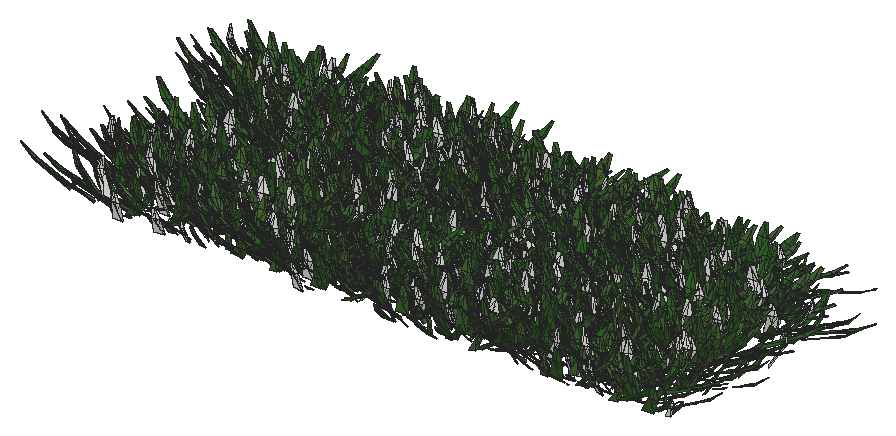
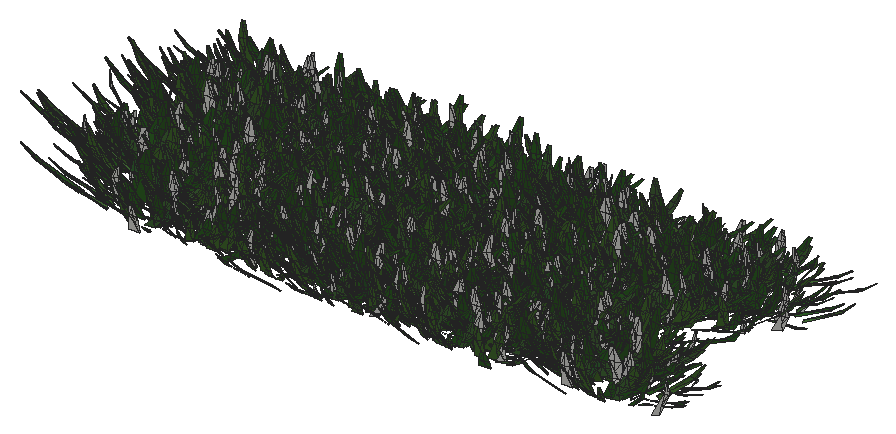
# SketchUp Ruby script. Lengths in inches.
U = 1.inch
M = Sketchup.active_model
def pt(a) = Geom::Point3d.new(a.map { |v| v * U })
def face(e, loops, mat)
  f = e.add_face(loops[0].map { |a| pt(a) })
  loops[1..].each { |l| e.add_face(l.map { |a| pt(a) }).erase! }
  f.material = f.back_material = mat if mat
  f
end
# faces: each face lists its corners as indices into pts; further lists are holes
def faces(e, pts, list, mat = nil) = list.each { |f| face(e, (f[0].is_a?(Array) ? f : [f]).map { |l| l.map { |i| pts[i] } }, mat) }
# xy, xz, yz: faces in a plane at the given z, y or x. An outline is a flat list of corners, or four numbers for a rectangle; further outlines are holes
def ring(l) = l.size == 4 ? [[l[0], l[1]], [l[2], l[1]], [l[2], l[3]], [l[0], l[3]]] : l.each_slice(2).to_a
def flat(e, list, mat, &to3) = list.each { |f| face(e, (f[0].is_a?(Array) ? f : [f]).map { |l| ring(l).map { |u, v| to3.(u, v) } }, mat) }
def xy(e, z, list, mat = nil) = flat(e, list, mat) { |x, y| [x, y, z] }
def xz(e, y, list, mat = nil) = flat(e, list, mat) { |x, z| [x, y, z] }
def yz(e, x, list, mat = nil) = flat(e, list, mat) { |y, z| [x, y, z] }
def lines(e, pts, list) = list.each { |a, b| e.add_line(pt(pts[a]), pt(pts[b])) }
# prism: a flat outline (further loops are holes) pulled along v
def prism(e, loops, v, mat = nil)
  f = face(e, loops, mat); d = Geom::Vector3d.new(v.map { |x| x * U })
  f.pushpull(f.normal.samedirection?(d) ? d.length : -d.length)
end
def box(e, o, s, mat = nil) = prism(e, [[o, [o[0] + s[0], o[1], o[2]], [o[0] + s[0], o[1] + s[1], o[2]], [o[0], o[1] + s[1], o[2]]]], [0, 0, s[2]], mat)
def at(x, y, z, deg = 0) = Geom::Transformation.translation(pt([x, y, z])) * Geom::Transformation.rotation(ORIGIN, Z_AXIS, deg.degrees)
def axes(o, x, y, z) = Geom::Transformation.new([*x, 0, *y, 0, *z, 0, *pt(o).to_a, 1])
def part(name) = M.definitions.add(name)
# library, detail: a bought-in or finely detailed component or shape, given as its bounding box
def library(name, o, s) = part(name).tap { |d| box(d.entities, o, s) }
def detail(e, o, s) = box(e.add_group.entities, o, s)
def put(e, d, t, mat = nil) = e.add_instance(d, t).tap { |i| i.material = mat if mat }
def group(e, t, mat = nil) = e.add_group.tap { |g| g.transformation = t; g.material = mat if mat }.entities
root = M.entities
M.materials.add("Material82").color = [68, 110, 58]
M.materials.add("Material83").color = [48, 90, 38]
M.materials.add("Material84").color = [68, 110, 48]
M.materials.add("Material85").color = [48, 90, 48]
M.materials.add("Material86").color = [58, 110, 58]
M.materials.add("Material87").color = [58, 90, 38]
M.materials.add("Material88").color = [68, 100, 58]
M.materials.add("Material89").color = [48, 100, 38]
c1 = part("grass00")
p = [[-0.6875,0.15,0],[-0.56,0.08,5.52],[-0.04,0.03,2.76],[0.48,-0.02,0],[0.35,-0.02,5.52],[-0.1,-0.14,5.52],
  [-0.12,0.65,8.37],[-0.42,0.65,8.37]]
faces(c1.entities,p,[[0,1,2,3],[3,2,4],[1,5,2],[5,4,2],[1,6,5],[4,5,6],[7,6,1]])
c2 = part("Group16\#1")
put(c2.entities,c1,axes([1.44,-0.61,-0.01],[0.05352,0.12609,0],[-0.10704,0.04543,0.07239],[0.06664,-0.02828,0.11628]),"Material85")
put(c2.entities,c1,axes([0.76,-0.15,-0.01],[0.04676,0.24062,0],[-0.23162,0.04501,0.06642],[0.0652,-0.01267,0.23595]),"Material82")
put(c2.entities,c1,axes([0.79,0.01,-0.01],[-0.00606,0.34651,0],[-0.34381,-0.00602,0.0432],[0.04319,0.00076,0.34386]))
put(c2.entities,c1,axes([1,0.23,-0.01],[-0.07192,0.31144,0],[-0.28722,-0.06632,0.1236],[0.12043,0.02781,0.29478]),"Material84")
put(c2.entities,c1,axes([1.66,0.77,-0.01],[-0.13828,0.29651,0],[-0.21551,-0.1005,0.22471],[0.20365,0.09498,0.23779]),"Material89")
put(c2.entities,c1,axes([0.6875,0.52,-0.01],[-0.18126,0.24051,0],[-0.22746,-0.17142,0.09788],[0.07817,0.05891,0.28481]),"Material84")
put(c2.entities,c1,axes([0.68,0.78,-0.01],[-0.215,0.18688,0],[-0.12385,-0.14248,0.21334],[0.13995,0.16101,0.18878]),"Material82")
put(c2.entities,c1,axes([0.56,1,-0.01],[-0.13756,0.07624,0],[-0.06159,-0.11112,0.0927],[0.04494,0.08108,0.12705]),"Material84")
put(c2.entities,c1,axes([0.2,0.64,-0.01],[-0.23729,0.07254,0],[-0.05711,-0.18681,0.153],[0.04473,0.14632,0.19535]),"Material89")
put(c2.entities,c1,axes([0.0625,0.72,-0.01],[-0.28874,0.02525,0],[-0.02179,-0.24916,0.14647],[0.01276,0.14591,0.25012]),"Material82")
put(c2.entities,c1,axes([-0.08,0.62,-0.01],[-0.34089,-0.04187,0],[0.03255,-0.26504,0.216],[-0.02633,0.21439,0.26703]),"Material89")
put(c2.entities,c1,axes([-0.34,0.98,-0.01],[-0.14314,-0.0493,0],[0.04397,-0.12769,0.06843],[-0.02228,0.0647,0.13505]),"Material89")
put(c2.entities,c1,axes([-0.87,1.45,-0.01],[-0.23488,-0.14114,0],[0.13761,-0.22901,0.06087],[-0.03135,0.05217,0.26717]))
put(c2.entities,c1,axes([-0.72,0.77,-0.01],[-0.14208,-0.13251,0],[0.07209,-0.0773,0.16301],[-0.11118,0.11922,0.1057]),"Material89")
put(c2.entities,c1,axes([-0.62,0.43,-0.01],[-0.14845,-0.21203,0],[0.18654,-0.13061,0.12304],[-0.10079,0.07057,0.22772]),"Material82")
put(c2.entities,c1,axes([-0.68,0.29,-0.01],[-0.13639,-0.32136,0],[0.31723,-0.13464,0.05579],[-0.05136,0.0218,0.34462]),"Material83")
put(c2.entities,c1,axes([-0.64,0.125,-0.01],[-0.0458,-0.23569,0],[0.22124,-0.043,0.08276],[-0.08124,0.01579,0.22538]),"Material86")
put(c2.entities,c1,axes([-1.6,-0.03,-0.01],[0.00576,-0.32897,0],[0.27526,0.00482,0.18018],[-0.18015,-0.00315,0.2753]),"Material84")
put(c2.entities,c1,axes([-1.36,-0.31,-0.01],[0.05718,-0.24765,0],[0.18172,0.04196,0.17267],[-0.16825,-0.03885,0.1865]),"Material89")
put(c2.entities,c1,axes([-1.54,-0.72,-0.01],[0.06537,-0.14017,0],[0.13555,0.06321,0.03939],[-0.0357,-0.01665,0.14956]))
put(c2.entities,c1,axes([-1.19,-0.9,-0.01],[0.09597,-0.12735,0],[0.11214,0.08451,0.07557],[-0.06035,-0.04548,0.14042]),"Material88")
put(c2.entities,c1,axes([-0.47,-0.54,-0.01],[0.11588,-0.10072,0],[0.0618,0.0711,0.12124],[-0.07953,-0.0915,0.0942]))
put(c2.entities,c1,axes([-0.47,-0.84,-0.01],[0.11927,-0.0661,0],[0.06603,0.11913,0.00646],[-0.00313,-0.00565,0.13621]),"Material84")
put(c2.entities,c1,axes([-0.38,-1.24,-0.01],[0.28037,-0.08571,0],[0.0618,0.20215,0.20315],[-0.05939,-0.19428,0.21139]),"Material88")
put(c2.entities,c1,axes([-0.06,-0.66,-0.01],[0.22719,-0.01987,0],[0.01247,0.14255,0.17758],[-0.01547,-0.17691,0.1431]),"Material87")
put(c2.entities,c1,axes([0.11,-0.89,-0.01],[0.14882,0.01828,0],[-0.01058,0.08611,0.12229],[0.01491,-0.12138,0.08676]),"Material85")
put(c2.entities,c1,axes([0.25,-0.72,-0.01],[0.20481,0.07053,0],[-0.06206,0.18022,0.10291],[0.03351,-0.0973,0.1906]),"Material85")
put(c2.entities,c1,axes([0.85,-1.42,-0.01],[0.16481,0.09904,0],[-0.09472,0.15762,0.05616],[0.02893,-0.04814,0.18389]),"Material84")
put(c2.entities,c1,axes([1.01,-1.09,-0.01],[0.21858,0.20385,0],[-0.17495,0.1876,0.15339],[0.10462,-0.11218,0.25652]),"Material89")
put(c2.entities,c1,axes([1.01,-0.71,-0.01],[0.08733,0.12473,0],[-0.06445,0.04512,0.13037],[0.1068,-0.07477,0.07867]),"Material85")
c3 = part("Group15\#1")
put(c3.entities,c2,at(0,0,0))
c4 = part("3darcstudiotree_grass00\#1")
put(c4.entities,c3,at(0,0,0))
put(root,c4,axes([1866.09,997.54,-29.74],[3.63959,0.40285,0],[-0.8944,1.25675,-0.00495],[-0.00749,0.01053,1.38942]))
put(root,c4,axes([1827.97,997.18,-29.74],[-3.14741,0.41412,0],[-1.12782,-1.33315,-0.01591],[-0.02767,-0.03271,1.46774]))
put(root,c4,axes([1850.34,997.39,-29.74],[-3.08585,0.75112,0],[-1.75968,-1.12437,-0.03387],[-0.09597,-0.06132,1.3548]))
put(root,c4,axes([1842.99,998.27,-29.74],[3.37216,0.16863,0],[-0.47809,1.48691,-0.01144],[-0.0086,0.02673,1.7012]))
put(root,c4,axes([1881.56,998.54,-29.74],[4.62364,0.41674,0],[-0.83657,1.44354,-0.00333],[-0.00361,0.00623,1.36941]))
put(root,c4,axes([1839.99,998.41,-29.74],[3.38325,1.26435,0],[-2.73925,1.14001,-0.00751],[-0.0314,0.01307,1.8142]))
put(root,c4,axes([1832.05,998.28,-29.74],[-3.54635,0.32604,0],[-1.06041,-1.79388,-0.06463],[-0.05576,-0.09432,1.33032]))
put(root,c4,axes([1859.83,998.95,-29.74],[-1.14276,-1.73672,0],[3.49011,-0.35717,-0.03225],[0.18285,-0.01871,1.58326]))
put(root,c4,axes([1878.23,999.05,-29.74],[3.63873,-0.8009,0],[1.86273,1.31624,-0.03495],[0.11311,0.07993,1.90256]))
put(root,c4,axes([1887.55,999.17,-29.74],[-1.8058,1.22943,0],[-3.0103,-0.68768,-0.02138],[-0.11593,-0.02648,1.63406]))
put(root,c4,axes([1866.27,999.67,-29.74],[-1.39646,-1.43145,0],[3.7454,-0.56828,-0.0371],[0.22587,-0.03427,1.96201]))
put(root,c4,axes([1853.81,999.49,-29.74],[-3.39608,-0.38473,0],[1.21289,-1.66516,-0.05258],[0.08123,-0.11153,1.84274]))
put(root,c4,axes([1871.78,999.74,-29.74],[-2.82588,-0.78458,0],[2.18733,-1.22531,-0.03828],[0.15336,-0.08591,1.98208]))
put(root,c4,axes([1847.45,999.59,-29.74],[-4.11359,0.33172,0],[-0.73599,-1.4195,-0.0347],[-0.04072,-0.07853,1.61275]))
put(root,c4,axes([1848.125,1000.4,-29.74],[2.00643,-1.16557,0],[2.7626,0.73963,-0.03969],[0.18592,0.04978,1.41714]))
put(root,c4,axes([1845.375,1000.67,-29.74],[-0.92987,-1.7368,0],[3.78348,-0.31505,-0.00703],[0.03581,-0.00298,1.50812]))
put(root,c4,axes([1881.77,1000.76,-29.74],[2.37064,0.94684,0],[-3.28047,1.27743,-0.04002],[-0.15051,0.05861,1.82631]))
put(root,c4,axes([1870.7,1001.11,-29.74],[-0.85576,-1.5606,0],[4.52661,-0.38605,-0.05631],[0.21879,-0.01866,1.37991]))
put(root,c4,axes([1831.39,1000.78,-29.74],[-3.5543,0.89209,0],[-1.79933,-1.11498,-0.04609],[-0.16829,-0.10428,1.7083]))
put(root,c4,axes([1860.6,1000.94,-29.74],[-4.19905,0.34301,0],[-0.96105,-1.82979,-0.05761],[-0.05651,-0.10759,1.71741]))
put(root,c4,axes([1865.51,1001.26,-29.74],[1.4538,1.50227,0],[-4.10712,0.61817,-0.00597],[-0.03083,0.00464,1.82255]))
put(root,c4,axes([1855.41,1001.8,-29.74],[3.76801,-0.42175,0],[1.14915,1.59678,-0.03157],[0.04846,0.06733,1.77323]))
put(root,c4,axes([1876.09,1001.65,-29.74],[-2.807,-0.90771,0],[2.30635,-1.10925,-0.04795],[0.15506,-0.07458,1.39039]))
put(root,c4,axes([1826.77,1001.8125,-29.74],[3.03313,0.50579,0],[-1.37798,1.28522,-0.04149],[-0.11611,0.10829,1.90578]))
put(root,c4,axes([1837.0625,1001.6875,-29.74],[0.41174,1.83159,0],[-3.96576,0.13865,-0.0152],[-0.08151,0.00285,1.60635]))
put(root,c4,axes([1826.7,1002.9375,-29.74],[4.0409,0.57443,0],[-1.45336,1.59011,-0.05978],[-0.09434,0.10321,1.49495]))
put(root,c4,axes([1866.85,1003.17,-29.74],[3.28196,0.81984,0],[-2.45781,1.53025,-0.01012],[-0.02495,0.01554,1.58691]))
put(root,c4,axes([1830.57,1002.9,-29.74],[-4.1133,-0.05921,0],[0.15009,-1.6218,-0.04384],[0.00865,-0.09349,1.66887]))
put(root,c4,axes([1886.63,1003.15,-29.74],[1.90217,1.207,0],[-3.00756,0.73717,-0.00184],[-0.00944,0.00231,1.60144]))
put(root,c4,axes([1849.4,1003.25,-29.74],[3.28108,0.9921,0],[-2.06723,1.06332,-0.03117],[-0.09708,0.04994,1.30357]))
put(root,c4,axes([1838.28,1003.66,-29.74],[1.64327,-1.14246,0],[4.09949,0.91708,-0.03953],[0.17253,0.0386,1.77239]))
put(root,c4,axes([1884.14,1003.49,-29.74],[2.92133,1.34194,0],[-2.9494,0.99861,-0.03135],[-0.14252,0.04825,1.74596]))
put(root,c4,axes([1842.74,1003.95,-29.74],[1.00632,-1.60929,0],[3.83281,0.37276,-0.00763],[0.0458,0.00445,1.82848]))
put(root,c4,axes([1854.36,1004.0625,-29.74],[3.61578,-1.02121,0],[2.66994,1.47029,-0.04389],[0.14306,0.07878,1.92393]))
put(root,c4,axes([1876.11,1003.79,-29.74],[2.97603,0.7742,0],[-2.07464,1.24033,-0.03997],[-0.14341,0.08574,1.84008]))
put(root,c4,axes([1861.24,1004.14,-29.74],[0.12061,-1.58998,0],[4.18389,0.04936,-0.01737],[0.08566,0.00101,1.54781]))
put(root,c4,axes([1872.79,1004.12,-29.74],[-1.60743,-1.14355,0],[3.95374,-0.86436,-0.00731],[0.03731,-0.00816,1.97847]))
put(root,c4,axes([1875.15,1004.83,-29.74],[3.2807,-0.61041,0],[1.81668,1.51857,-0.02435],[0.05518,0.04613,1.69455]))
put(root,c4,axes([1885.93,1005.08,-29.74],[3.15887,-0.80876,0],[1.92191,1.16751,-0.02789],[0.09845,0.05981,1.71527]))
put(root,c4,axes([1854.49,1005.05,-29.74],[-0.00326,-1.3732,0],[3.39922,-0.00125,-0.0371],[0.2688,-0.0001,1.84609]))
put(root,c4,axes([1870.72,1004.89,-29.74],[-3.59941,0.74413,0],[-1.52837,-1.14979,-0.02232],[-0.06679,-0.05025,1.59039]))
put(root,c4,axes([1838.08,1005.21,-29.74],[0.9145,1.75116,0],[-3.69114,0.2998,-0.03105],[-0.20233,0.01643,1.87912]))
put(root,c4,axes([1832.09,1005.54,-29.74],[-2.34222,-1.01748,0],[3.28821,-1.17726,-0.05879],[0.21723,-0.07777,1.66118]))
put(root,c4,axes([1827.74,1005.81,-29.74],[1.55138,-1.30688,0],[2.99369,0.55272,-0.04141],[0.29892,0.05519,1.97468]))
put(root,c4,axes([1866.78,1005.58,-29.74],[-1.85188,1.07885,0],[-3.29338,-0.87924,-0.00267],[-0.01201,-0.00321,1.62102]))
put(root,c4,axes([1843.28,1006.01,-29.74],[3.42011,0.99957,0],[-2.24279,1.19352,-0.03152],[-0.09807,0.05219,1.47514]))
put(root,c4,axes([1883.21,1005.85,-29.74],[-3.64839,-0.0594,0],[0.18827,-1.79867,-0.05407],[0.01098,-0.10487,1.68402]))
put(root,c4,axes([1847.11,1006.3,-29.74],[0.26665,1.72733,0],[-3.78087,0.09078,-0.02381],[-0.14887,0.00357,1.77807]))
put(root,c4,axes([1860.79,1006.3,-29.74],[-0.34365,1.56469,0],[-3.45908,-0.11816,-0.04948],[-0.26965,-0.00921,1.42361]))
put(root,c4,axes([1854.24,1006.94,-29.74],[-0.07574,-1.47303,0],[4.38332,-0.03505,-0.05384],[0.21677,-0.00173,1.32332]))
put(root,c4,axes([1839.2,1007.13,-29.74],[0.23576,-1.73441,0],[4.70751,0.09952,-0.00697],[0.03732,0.00079,1.89407]))
put(root,c4,axes([1886.76,1007.0625,-29.74],[-3.60106,0.31713,0],[-0.9107,-1.60836,-0.00123],[-0.0017,-0.003,1.99006]))
put(root,c4,axes([1869.49,1007.84,-29.74],[-0.83235,-1.28841,0],[3.31595,-0.33318,-0.03395],[0.19708,-0.0198,1.53644]))
put(root,c4,axes([1861.11,1007.83,-29.74],[4.55756,-0.02191,0],[0.04205,1.36049,-0.04731],[0.00354,0.1146,1.58849]))
put(root,c4,axes([1850.85,1007.71,-29.74],[-4.36692,-0.69342,0],[1.6396,-1.60594,-0.01703],[0.03175,-0.0311,1.64249]))
put(root,c4,axes([1883.8,1007.85,-29.74],[-4.39804,-0.22301,0],[0.45888,-1.40747,-0.03967],[0.03344,-0.10258,1.78282]))
put(root,c4,axes([1866.33,1007.92,-29.74],[-3.9934,-0.49353,0],[1.06998,-1.34652,-0.00157],[0.00241,-0.00304,1.37913]))
put(root,c4,axes([1845.58,1008.24,-29.74],[-2.16285,-1.07783,0],[3.1191,-0.97346,-0.00813],[0.02825,-0.00882,1.32168]))
put(root,c4,axes([1833.04,1008.125,-29.74],[-3.56597,0.54096,0],[-1.21057,-1.24113,-0.01112],[-0.02689,-0.02757,1.70172]))
put(root,c4,axes([1877.73,1008.49,-29.74],[-3.12571,-0.7496,0],[2.43282,-1.57777,-0.06276],[0.13907,-0.09019,1.49667]))
put(root,c4,axes([1867.52,1009.44,-29.74],[2.80724,-1.17226,0],[3.04027,1.13235,-0.05261],[0.16943,0.06311,1.38839]))
put(root,c4,axes([1871.84,1009.32,-29.74],[3.98724,0.20884,0],[-0.61603,1.82924,-0.05242],[-0.03685,0.10943,1.87281]))
put(root,c4,axes([1843.34,1009.29,-29.74],[-2.49579,-0.85332,0],[2.16334,-0.98408,-0.00893],[0.04692,-0.02134,1.98619]))
put(root,c4,axes([1877.34,1009.21,-29.74],[-0.65898,1.54379,0],[-3.85922,-0.25621,-0.04712],[-0.21087,-0.014,1.33133]))
put(root,c4,axes([1831.5,1009.15,-29.74],[-1.96915,1.54328,0],[-4.06414,-0.80652,-0.00338],[-0.01619,-0.00321,1.82725]))
put(root,c4,axes([1886.54,1010.09,-29.74],[-0.6545,-1.64207,0],[4.59681,-0.28496,-0.0381],[0.20859,-0.01293,1.93318]))
put(root,c4,axes([1853.21,1010.12,-29.74],[-3.35579,-1.19548,0],[2.90415,-1.2679,-0.0585],[0.2305,-0.10063,1.90866]))
put(root,c4,axes([1847.8,1009.94,-29.74],[1.02208,1.31259,0],[-4.10151,0.49672,-0.03259],[-0.17155,0.02078,1.77089]))
put(root,c4,axes([1858.75,1010.25,-29.74],[-1.37112,-1.31689,0],[3.73876,-0.60543,-0.04381],[0.2334,-0.0378,1.74465]))
put(root,c4,axes([1838.35,1009.94,-29.74],[1.28043,1.73979,0],[-3.30316,0.37809,-0.03743],[-0.19576,0.02241,1.40382]))
put(root,c4,axes([1880.29,1010.07,-29.74],[-1.11481,1.68554,0],[-3.85911,-0.39697,-0.04083],[-0.25467,-0.0262,1.92702]))
put(root,c4,axes([1884.06,1011.3,-29.74],[4.4065,0.29877,0],[-0.73465,1.68517,-0.00744],[-0.00712,0.01634,1.83611]))
put(root,c4,axes([1869.83,1011.46,-29.74],[-0.43709,-1.41781,0],[4.63894,-0.22243,-0.04217],[0.16902,-0.0081,1.41426]))
put(root,c4,axes([1877.95,1011.53,-29.74],[-2.31531,-0.95478,0],[2.79879,-1.05558,-0.03327],[0.10847,-0.04091,1.30962]))
put(root,c4,axes([1839,1011.8125,-29.74],[-3.49986,-0.57002,0],[1.44663,-1.38143,-0.04671],[0.11633,-0.11108,1.85324]))
put(root,c4,axes([1843.66,1011.56,-29.74],[-3.56783,-0.13568,0],[0.42403,-1.73414,-0.0118],[0.00459,-0.01877,1.34216]))
put(root,c4,axes([1860.35,1011.86,-29.74],[1.76415,1.1719,0],[-3.51067,0.82196,-0.05173],[-0.20066,0.04698,1.38038]))
put(root,c4,axes([1834.38,1012.2,-29.74],[3.28347,0.12106,0],[-0.38901,1.64106,-0.04931],[-0.02254,0.09507,1.538]))
put(root,c4,axes([1854.21,1011.93,-29.74],[-3.58969,-0.07657,0],[0.18796,-1.37056,-0.00522],[0.00152,-0.01105,1.40302]))
put(root,c4,axes([1849.03,1012.74,-29.74],[-2.85144,-1.16634,0],[2.50888,-0.95396,-0.03577],[0.14723,-0.05598,1.49339]))
put(root,c4,axes([1866.8125,1012.85,-29.74],[-3.70101,0.79314,0],[-2.22235,-1.61286,-0.04664],[-0.10432,-0.07571,1.63424]))
put(root,c4,axes([1859.79,1013.69,-29.74],[-2.51613,1.14478,0],[-2.79457,-0.95529,-0.04719],[-0.16752,-0.05727,1.30223]))
put(root,c4,axes([1834.37,1013.84,-29.74],[-3.8899,-0.78174,0],[2.11548,-1.63718,-0.02171],[0.04442,-0.03438,1.57387]))
put(root,c4,axes([1848.71,1014.18,-29.74],[-1.26006,-1.32624,0],[4.43512,-0.65537,-0.00645],[0.02239,-0.00331,1.31612]))
put(root,c4,axes([1837.18,1013.81,-29.74],[-3.55041,0.9087,0],[-2.02381,-1.22981,-0.02727],[-0.0752,-0.0457,1.41127]))
put(root,c4,axes([1870.96,1014.14,-29.74],[-2.86852,-0.72551,0],[1.94813,-1.19796,-0.01822],[0.05809,-0.03572,1.59761]))
put(root,c4,axes([1841.7,1014.48,-29.74],[-0.24051,-1.38856,0],[3.98568,-0.10737,-0.04502],[0.19517,-0.00526,1.30109]))
put(root,c4,axes([1876.94,1014.52,-29.74],[1.80555,1.12349,0],[-3.92794,0.98179,-0.01772],[-0.05919,0.0148,1.37883]))
put(root,c4,axes([1865.14,1014.75,-29.74],[3.1901,1.34772,0],[-3.0794,1.13365,-0.04297],[-0.19725,0.07262,1.98261]))
put(root,c4,axes([1855.05,1014.93,-29.74],[-3.3619,-0.88005,0],[2.60897,-1.55009,-0.03911],[0.08798,-0.05227,1.43856]))
put(root,c4,axes([1884.1,1014.74,-29.74],[-3.86294,0.12208,0],[-0.37038,-1.82279,-0.02116],[-0.00872,-0.04291,1.79229]))
put(root,c4,axes([1843,1016.09,-29.74],[4.22834,-0.67564,0],[1.61938,1.57623,-0.01357],[0.03127,0.03043,1.98263]))
put(root,c4,axes([1848.36,1015.97,-29.74],[0.22416,-1.4452,0],[4.13727,0.09981,-0.05271],[0.23324,0.00563,1.37729]))
put(root,c4,axes([1861.81,1016,-29.74],[-3.70247,-0.49757,0],[1.50858,-1.74588,-0.06303],[0.09341,-0.1081,1.61067]))
put(root,c4,axes([1832.375,1016.24,-29.74],[4.24476,0.21314,0],[-0.43337,1.34235,-0.04636],[-0.04216,0.1306,1.85211]))
put(root,c4,axes([1840.09,1016.7,-29.74],[4.08655,-0.74198,0],[1.4526,1.2443,-0.00355],[0.00912,0.00781,1.60125]))
put(root,c4,axes([1878.02,1016.23,-29.74],[-3.94904,-0.28889,0],[0.74698,-1.58808,-0.00704],[0.00779,-0.01657,1.86241]))
put(root,c4,axes([1884.17,1016.95,-29.74],[4.62049,-0.36242,0],[0.91883,1.82189,-0.02703],[0.02558,0.05072,1.71263]))
put(root,c4,axes([1869.26,1017.05,-29.74],[3.88367,-0.39615,0],[1.13822,1.73547,-0.04841],[0.06323,0.0964,1.77682]))
put(root,c4,axes([1865.86,1016.47,-29.74],[-1.78787,1.37846,0],[-3.47115,-0.7002,-0.05082],[-0.20934,-0.04223,1.35221]))
put(root,c4,axes([1887.54,1016.97,-29.74],[-1.11998,1.52641,0],[-4.36702,-0.49835,-0.06381],[-0.30025,-0.03426,1.66913]))
put(root,c4,axes([1828.11,1017.29,-29.74],[-0.77153,1.33479,0],[-3.28421,-0.29525,-0.03421],[-0.24787,-0.02228,1.87625]))
put(root,c4,axes([1852.62,1017.26,-29.74],[-1.26035,1.30994,0],[-3.37363,-0.50484,-0.03389],[-0.19382,-0.029,1.65454]))
put(root,c4,axes([1843.97,1017.86,-29.74],[3.74003,-0.3626,0],[0.86697,1.39078,-0.02888],[0.04393,0.07047,1.73467]))
put(root,c4,axes([1858.55,1018.03,-29.74],[3.65327,1.04493,0],[-2.10749,1.14596,-0.01189],[-0.03901,0.02121,1.50367]))
put(root,c4,axes([1883.85,1018.36,-29.74],[-2.13062,-1.66467,0],[3.82642,-0.7617,-0.02075],[0.09652,-0.01921,1.67433]))
put(root,c4,axes([1832.3,1018.52,-29.74],[-0.28709,-1.61704,0],[4.14071,-0.11434,-0.04142],[0.22933,-0.00633,1.72685]))
put(root,c4,axes([1878.75,1018.02,-29.74],[-2.45667,1.24552,0],[-3.48685,-1.06965,-0.01031],[-0.04097,-0.01257,1.66779]))
put(root,c4,axes([1885.9,1018.34,-29.74],[-4.37191,-0.09188,0],[0.22077,-1.63377,-0.04256],[0.01218,-0.09013,1.67228]))
put(root,c4,axes([1827.58,1019.15,-29.74],[4.14328,-0.46419,0],[1.00154,1.39037,-0.02465],[0.03463,0.04808,1.41248]))
put(root,c4,axes([1836.73,1018.78,-29.74],[1.12356,1.5327,0],[-3.46853,0.39546,-0.04889],[-0.25471,0.02904,1.46761]))
put(root,c4,axes([1869.36,1019.04,-29.74],[1.48622,1.27925,0],[-3.96463,0.71638,-0.00338],[-0.01448,0.00262,1.53978]))
put(root,c4,axes([1849.71,1019.39,-29.74],[-0.17296,-1.31916,0],[4.52056,-0.09218,-0.00424],[0.01978,-0.0004,1.58408]))
put(root,c4,axes([1865.13,1019.15,-29.74],[-3.91187,0.00169,0],[-0.00401,-1.44027,-0.04481],[-0.00031,-0.10997,1.70362]))
put(root,c4,axes([1852.88,1019.34,-29.74],[-3.17197,-0.90891,0],[2.49685,-1.35522,-0.03763],[0.13517,-0.07337,1.94544]))
put(root,c4,axes([1876.34,1020.04,-29.74],[-1.43959,-1.62411,0],[3.7168,-0.5124,-0.03865],[0.23963,-0.03303,1.9383]))
put(root,c4,axes([1866.61,1020.17,-29.74],[-3.49916,1.06741,0],[-2.60054,-1.32589,-0.05181],[-0.14447,-0.07366,1.45196]))
put(root,c4,axes([1831.85,1020.69,-29.74],[3.55843,0.77732,0],[-2.07504,1.47739,-0.02111],[-0.0608,0.04329,1.90804]))
put(root,c4,axes([1838.84,1020.63,-29.74],[2.41483,0.92576,0],[-3.06998,1.24547,-0.04673],[-0.14351,0.05822,1.45453]))
put(root,c4,axes([1855.71,1020.61,-29.74],[2.09185,1.03032,0],[-2.8732,0.90727,-0.01526],[-0.08429,0.02662,1.9517]))
put(root,c4,axes([1859.79,1021.46,-29.74],[3.21656,-1.06764,0],[2.25071,1.05463,-0.04982],[0.17505,0.08203,1.4295]))
put(root,c4,axes([1882.73,1020.76,-29.74],[-3.05865,1.0781,0],[-2.78611,-1.22937,-0.02716],[-0.07662,-0.03381,1.32671]))
put(root,c4,axes([1828.45,1020.83,-29.74],[-1.91367,1.54924,0],[-4.25661,-0.81775,-0.00711],[-0.02422,-0.00465,1.34501]))
put(root,c4,axes([1872.82,1021.04,-29.74],[-3.32772,0.28661,0],[-0.75668,-1.36642,-0.01018],[-0.01111,-0.02006,1.35975]))
put(root,c4,axes([1847.09,1021.3,-29.74],[-2.99545,-1.01525,0],[2.44315,-1.12112,-0.00129],[0.00439,-0.00201,1.46122]))
put(root,c4,axes([1844.99,1021.61,-29.74],[-2.35271,1.42324,0],[-3.1761,-0.81658,-0.00573],[-0.02769,-0.00712,1.63969]))
put(root,c4,axes([1839.28,1022.63,-29.74],[4.28624,-0.48224,0],[1.29741,1.79351,-0.04256],[0.05122,0.07081,1.55488]))
put(root,c4,axes([1871.34,1022.83,-29.74],[1.63817,-1.67164,0],[3.7967,0.57868,-0.011],[0.05001,0.00762,1.48653]))
put(root,c4,axes([1831.14,1022.85,-29.74],[3.65348,-0.50094,0],[1.24961,1.41744,-0.02118],[0.04225,0.04793,1.73224]))
put(root,c4,axes([1843.29,1023.11,-29.74],[2.15184,-1.02148,0],[3.44742,1.1295,-0.00974],[0.03611,0.01183,1.619]))
put(root,c4,axes([1865.25,1022.84,-29.74],[-3.74528,-0.54225,0],[1.29092,-1.38673,-0.02574],[0.04375,-0.047,1.38465]))
put(root,c4,axes([1859.37,1023.26,-29.74],[-0.8424,-1.2576,0],[4.34376,-0.45254,-0.01354],[0.07406,-0.00772,1.90468]))
put(root,c4,axes([1881.65,1022.86,-29.74],[-3.30618,0.81403,0],[-2.41899,-1.52802,-0.02972],[-0.07466,-0.04716,1.62371]))
put(root,c4,axes([1877.03,1023.03,-29.74],[-3.81782,0.15844,0],[-0.49654,-1.86087,-0.00853],[-0.00435,-0.0163,1.7318]))
put(root,c4,axes([1826.57,1023.76,-29.74],[3.09052,1.16305,0],[-2.75216,1.13741,-0.00767],[-0.03246,0.01341,1.8325]))
put(root,c4,axes([1854.28,1023.61,-29.74],[-3.78052,0.58265,0],[-1.19847,-1.20943,-0.02866],[-0.07958,-0.08031,1.88291]))
put(root,c4,axes([1847.8,1023.8,-29.74],[2.93363,1.22701,0],[-2.56818,0.95498,-0.02839],[-0.14721,0.05474,1.88589]))
put(root,c4,axes([1880.81,1024.94,-29.74],[3.83562,-0.64652,0],[1.50566,1.38929,-0.01454],[0.02594,0.02394,1.30369]))
put(root,c4,axes([1839.62,1024.48,-29.74],[0.63995,1.63517,0],[-3.50377,0.21327,-0.04631],[-0.28502,0.01735,1.65491]))
put(root,c4,axes([1872.84,1024.55,-29.74],[-0.30333,1.33059,0],[-3.40704,-0.1208,-0.0349],[-0.19211,-0.00681,1.41691]))
put(root,c4,axes([1865.17,1024.8,-29.74],[2.25108,1.29367,0],[-3.07657,0.83262,-0.0512],[-0.2098,0.05678,1.38975]))
put(root,c4,axes([1858.84,1025.05,-29.74],[3.43468,1.02641,0],[-2.59272,1.34938,-0.0181],[-0.04577,0.02382,1.34745]))
put(root,c4,axes([1855.28,1024.99,-29.74],[-2.81078,-0.75848,0],[2.18011,-1.25652,-0.01797],[0.04803,-0.02768,1.36964]))
put(root,c4,axes([1843.98,1025.14,-29.74],[2.54513,1.12368,0],[-2.54126,0.89522,-0.01423],[-0.07597,0.02676,1.82816]))
